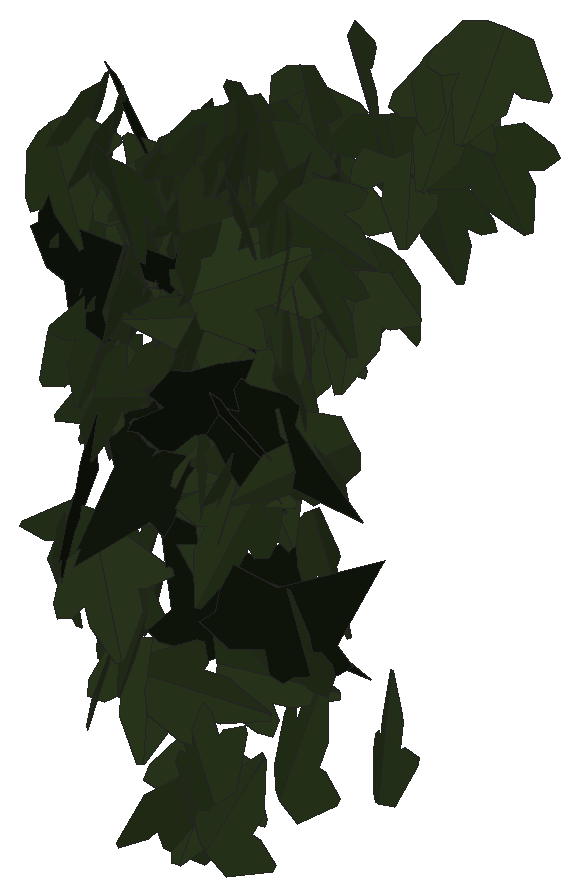
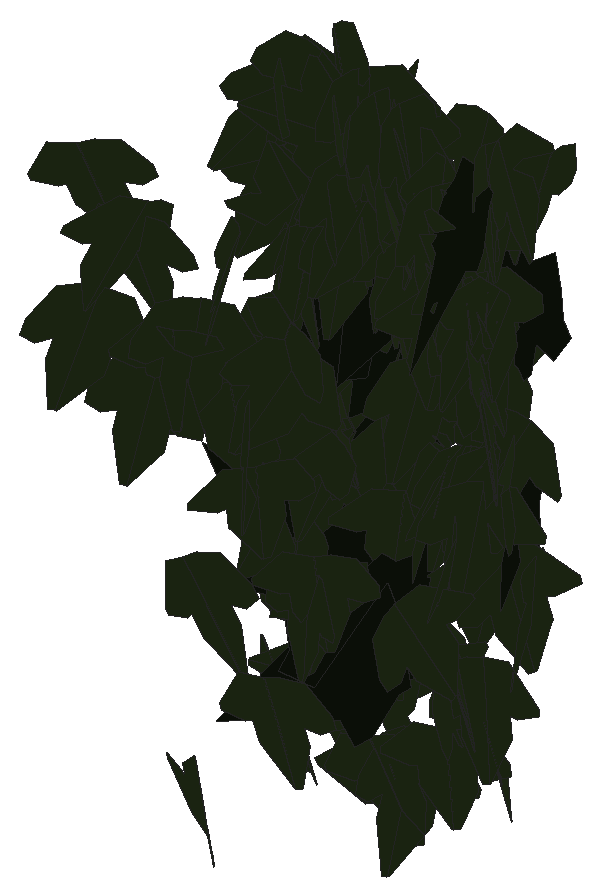
# SketchUp Ruby script. Lengths in inches.
U = 1.inch
M = Sketchup.active_model
def pt(a) = Geom::Point3d.new(a.map { |v| v * U })
def face(e, loops, mat)
  f = e.add_face(loops[0].map { |a| pt(a) })
  loops[1..].each { |l| e.add_face(l.map { |a| pt(a) }).erase! }
  f.material = f.back_material = mat if mat
  f
end
# faces: each face lists its corners as indices into pts; further lists are holes
def faces(e, pts, list, mat = nil) = list.each { |f| face(e, (f[0].is_a?(Array) ? f : [f]).map { |l| l.map { |i| pts[i] } }, mat) }
# xy, xz, yz: faces in a plane at the given z, y or x. An outline is a flat list of corners, or four numbers for a rectangle; further outlines are holes
def ring(l) = l.size == 4 ? [[l[0], l[1]], [l[2], l[1]], [l[2], l[3]], [l[0], l[3]]] : l.each_slice(2).to_a
def flat(e, list, mat, &to3) = list.each { |f| face(e, (f[0].is_a?(Array) ? f : [f]).map { |l| ring(l).map { |u, v| to3.(u, v) } }, mat) }
def xy(e, z, list, mat = nil) = flat(e, list, mat) { |x, y| [x, y, z] }
def xz(e, y, list, mat = nil) = flat(e, list, mat) { |x, z| [x, y, z] }
def yz(e, x, list, mat = nil) = flat(e, list, mat) { |y, z| [x, y, z] }
def lines(e, pts, list) = list.each { |a, b| e.add_line(pt(pts[a]), pt(pts[b])) }
# prism: a flat outline (further loops are holes) pulled along v
def prism(e, loops, v, mat = nil)
  f = face(e, loops, mat); d = Geom::Vector3d.new(v.map { |x| x * U })
  f.pushpull(f.normal.samedirection?(d) ? d.length : -d.length)
end
def box(e, o, s, mat = nil) = prism(e, [[o, [o[0] + s[0], o[1], o[2]], [o[0] + s[0], o[1] + s[1], o[2]], [o[0], o[1] + s[1], o[2]]]], [0, 0, s[2]], mat)
def at(x, y, z, deg = 0) = Geom::Transformation.translation(pt([x, y, z])) * Geom::Transformation.rotation(ORIGIN, Z_AXIS, deg.degrees)
def axes(o, x, y, z) = Geom::Transformation.new([*x, 0, *y, 0, *z, 0, *pt(o).to_a, 1])
def part(name) = M.definitions.add(name)
# library, detail: a bought-in or finely detailed component or shape, given as its bounding box
def library(name, o, s) = part(name).tap { |d| box(d.entities, o, s) }
def detail(e, o, s) = box(e.add_group.entities, o, s)
def put(e, d, t, mat = nil) = e.add_instance(d, t).tap { |i| i.material = mat if mat }
def group(e, t, mat = nil) = e.add_group.tap { |g| g.transformation = t; g.material = mat if mat }.entities
root = M.entities
M.materials.add("efeu1").color = [18, 25, 13]
M.materials.add("efeu2").color = [43, 57, 29]
c1 = part("ivyleaf_10")
p = [[0,0.5,-0.03],[-0.0625,2.02,-0.43],[-0.19,2.01,-0.46],[-0.54,1.05,-0.29],[-0.52,0.625,-0.18],[-0.83,0.76,-0.28],
  [-1.16,0.64,-0.33],[-1.15,0.33,-0.24],[-0.77,-0.39,0.02],[-0.3,-0.51,0.16],[0.04,-0.48,0.23],[-0.02,2.01,-0.4375],
  [-0.06,2.01,-0.43],[0.04,-0.49,0.23],[0.67,-0.49,0.14],[1.38,0.36,-0.2],[1.375,0.51,-0.24],[0.81,0.65,-0.19],
  [0.62,0.59,-0.15],[0.6,1.09,-0.28],[0.5,1.23,-0.31]]
faces(c1.entities,p,[[0,1,2,3,4,5,6,7,8,9,10],[11,12,0,13,14,15,16,17,18,19,20]],"efeu2")
c2 = part("ivyleaf_9")
p = [[1.54,2.16,1.25],[1.36,2.04,1.19],[-0.21,0.99,0.68],[-0.71,1.11,0.82],[-0.85,0.86,0.67],[-0.8,0.17,0.21],
  [-0.9,-0.01,0.1],[-0.67,-0.16,-0.02],[-0.08,-0.08,-0.05],[-0.03,-0.6,-0.4],[0.65,-0.88,-0.66],[0.83,-0.6,-0.49],
  [1.29,-0.42,-0.43],[1.8125,-0.07,-0.26],[1.21,0.44,0.15]]
faces(c2.entities,p,[[0,1,2,3,4,5,6,7,8,9,10,11,12,13,14]],"efeu1")
put(root,c1,axes([526.73,137.66,179.65],[0.34492,-0.55655,-0.19979],[-0.07334,0.18925,-0.65379],[0.58676,0.35081,0.03573]))
put(root,c1,axes([526.55,141.41,178.74],[0.59733,0.31347,-0.01678],[-0.01478,-0.00794,-0.67459],[-0.31357,0.59751,-0.00017]))
put(root,c1,axes([526.68,142.2,177.14],[0.6762,0.08427,-0.10291],[-0.10981,0.05281,-0.6783],[-0.07506,0.68194,0.06524]))
put(root,c1,axes([526.32,137.64,178.37],[0.22626,-0.32432,0.5422],[0.5291,-0.21748,-0.35088],[0.34528,0.54578,0.18237]))
put(root,c1,axes([526.96,136.28,176.09],[-0.253,0.3315,0.61469],[-0.38291,0.48091,-0.41696],[-0.58405,-0.45889,0.00709]))
put(root,c1,axes([526.73,137.78,178.06],[-0.4918,-0.46006,-0.10041],[0.12139,0.01642,-0.66977],[0.45497,-0.50167,0.07016]))
put(root,c1,axes([526.75,137.6,180.96],[0.06524,0.49402,0.48223],[-0.14861,0.48307,-0.47477],[-0.67417,-0.05868,0.15132]))
put(root,c1,axes([526.76,137.09,182.98],[0.15346,-0.69055,0.08481],[0.03468,-0.07915,-0.7072],[0.69488,0.15646,0.01657]))
put(root,c1,axes([526.82,141.39,178.37],[-0.62666,0.24212,0.03133],[-0.07654,-0.11287,-0.65856],[-0.23184,-0.6172,0.13272]))
put(root,c1,axes([526.55,137.1875,178.94],[-0.59271,-0.09398,-0.31926],[0.33268,-0.18537,-0.56305],[-0.00921,-0.6472,0.20763]))
put(root,c1,axes([526.95,137.45,175.16],[-0.65274,-0.09316,0.14039],[-0.13169,-0.06832,-0.65761],[0.10511,-0.66416,0.04796]))
put(root,c1,axes([526.91,139.04,176.77],[-0.16863,-0.55856,0.33637],[-0.03052,-0.34029,-0.58037],[0.65131,-0.16056,0.05989]))
put(root,c1,axes([526.89,137.52,181.05],[-0.2547,-0.64705,0.0378],[0.01176,-0.04522,-0.69483],[0.64804,-0.25349,0.02747]))
put(root,c1,axes([526.84,137.56,180.46],[0.20743,-0.65308,0.08528],[0.04003,-0.07674,-0.68508],[0.65741,0.21074,0.01481]))
put(root,c1,axes([527.0625,136.78,176.48],[-0.49027,-0.429,0.20414],[-0.13677,-0.15347,-0.65101],[0.45498,-0.50841,0.02427]))
put(root,c1,axes([526.79,138.34,177.59],[-0.29412,0.56067,-0.22412],[0.06235,-0.21976,-0.63159],[-0.60058,-0.29739,0.04419]))
put(root,c2,axes([526.875,137.77,182.61],[0.61826,-0.11639,-0.51976],[-0.4988,0.15278,-0.62754],[0.18681,0.79313,0.04461]))
put(root,c1,axes([526.79,136.36,182.55],[0.08652,0.72593,0.09804],[0.01904,0.09646,-0.73103],[-0.73227,0.08827,-0.00742]))
put(root,c1,axes([527,137.21,174.38],[0.38779,-0.55151,0.00364],[0.0023,-0.00284,-0.6742],[0.55152,0.3878,0.00025]))
put(root,c1,axes([527.37,137.79,177.8],[-0.54902,0.02235,-0.40135],[-0.40086,0.02003,0.54947],[0.02987,0.67978,-0.00299]))
put(root,c1,axes([527.1,137.05,182.73],[0.13063,-0.67134,-0.19616],[-0.03098,0.1938,-0.68391],[0.69873,0.13411,0.00635]))
put(root,c2,axes([526.62,136.75,180.27],[-0.08717,0.03371,0.78745],[0.44244,-0.65356,0.07696],[0.65227,0.44781,0.05303]))
put(root,c1,axes([527.11,137.1,179.79],[-0.09112,-0.67476,0.2638],[0.04855,-0.27097,-0.67632],[0.72286,-0.06685,0.07868]))
put(root,c2,axes([527.5,135.88,177.56],[-0.10562,0.10538,-0.81586],[-0.70882,0.4058,0.14418],[0.4175,0.71562,0.03838]))
put(root,c1,axes([527.22,137.16,181.21],[-0.53677,0.44477,0.03747],[-0.09582,-0.05758,-0.68909],[-0.43594,-0.53498,0.10532]))
put(root,c1,axes([527.17,137.8,175.63],[0.40583,-0.54322,0.02309],[0.01224,-0.01968,-0.67808],[0.54358,0.40601,-0.00197]))
put(root,c1,axes([527.17,137.51,181.125],[0.38421,-0.57202,-0.11484],[0.02053,0.15067,-0.68183],[0.58307,0.37162,0.09968]))
put(root,c1,axes([527.28,137.51,180.91],[0.546,-0.39262,-0.12601],[-0.1101,0.06268,-0.67238],[0.39737,0.55684,-0.01316]))
put(root,c1,axes([527.18,137.51,178.33],[-0.25362,-0.58125,-0.24503],[0.17351,0.18962,-0.62941],[0.60645,-0.29733,0.07761]))
put(root,c1,axes([527.67,137.58,181.76],[-0.4948,0.16819,0.44755],[-0.47688,-0.21967,-0.44469],[0.03418,-0.62998,0.27454]))
put(root,c1,axes([527.22,136.88,178.59],[-0.06189,-0.32946,-0.66162],[0.1774,0.63791,-0.33424],[0.71751,-0.18613,0.02557]))
put(root,c1,axes([527.1875,140.28,177.8125],[0.13331,0.65307,0.13137],[-0.00807,0.13555,-0.66565],[-0.6661,0.12906,0.03436]))
put(root,c1,axes([527.34,137.43,180.99],[-0.47146,0.51453,0.03959],[-0.03584,0.02085,-0.69775],[-0.5148,-0.47266,0.01232]))
put(root,c1,axes([527.27,137.69,180.78],[0.43151,0.50537,0.17621],[-0.00926,0.23337,-0.64661],[-0.53513,0.40347,0.15329]))
put(root,c1,axes([527.31,137.67,175.05],[0.16404,-0.57953,0.34818],[0.16922,-0.31168,-0.59851],[0.65456,0.22582,0.06747]))
put(root,c1,axes([527.46,137.33,180.51],[-0.01063,-0.70751,-0.00159],[0.00785,0.00147,-0.70754],[0.70746,-0.01064,0.00783]))
put(root,c1,axes([527.56,136.83,181.78],[-0.61387,0.27502,0.1835],[-0.16992,0.06952,-0.67263],[-0.28361,-0.63693,0.00582]))
put(root,c1,axes([527.53,137.39,181.24],[-0.17121,0.65872,0.16593],[-0.18514,0.1194,-0.665],[-0.65358,-0.20637,0.1449]))
put(root,c1,axes([527.62,136.93,181.9375],[-0.6839,-0.15676,0.04606],[-0.02555,-0.09317,-0.69647],[0.16137,-0.67908,0.08493]))
put(root,c1,axes([527.5,137.71,178.03],[-0.27325,0.62473,0.06912],[-0.02884,0.06282,-0.68187],[-0.62788,-0.27477,0.00124]))
put(root,c1,axes([527.57,137.5625,178.33],[-0.46744,0.48932,0.07753],[-0.05575,0.05397,-0.6767],[-0.49228,-0.47074,0.00301]))
put(root,c1,axes([527.4,140.95,181.3125],[-0.52133,-0.29503,-0.33284],[0.30593,0.13437,-0.5983],[0.32284,-0.60375,0.02949]))
put(root,c1,axes([527.43,137.53,174.08],[0.63628,0.29088,0.02502],[0.01821,0.02033,-0.69954],[-0.29138,0.63645,0.01091]))
put(root,c1,axes([527.6875,137.52,181.07],[-0.44649,-0.52236,-0.09133],[0.05124,0.07633,-0.6871],[0.5278,-0.4493,-0.01055]))
put(root,c1,axes([527.59,141.41,179.76],[0.44109,0.51607,-0.0565],[-0.0262,-0.05192,-0.67875],[-0.51849,0.44165,-0.01377]))
put(root,c1,axes([527.75,141.29,180.46],[0.18437,-0.56899,-0.32951],[-0.01701,0.33797,-0.59313],[0.6573,0.16834,0.07707]))
put(root,c1,axes([527.75,137.46,182.05],[-0.09166,-0.68778,-0.07675],[0.09267,0.06452,-0.6889],[0.68582,-0.10064,0.08283]))
put(root,c1,axes([527.59,136.32,176.2],[0.39292,0.54626,0.12166],[0.06463,0.10336,-0.67285],[-0.5559,0.39813,0.00776]))
put(root,c1,axes([527.48,140.87,181.74],[0.60239,-0.14425,0.30188],[0.32288,0.08776,-0.60237],[0.08766,0.66806,0.14431]))
put(root,c1,axes([527.69,137.48,181.51],[0.46198,0.50867,0.01464],[-0.00205,0.02164,-0.68696],[-0.50887,0.46171,0.01607]))
put(root,c1,axes([528.01,142.12,178.44],[0.5981,-0.03936,-0.35907],[-0.34125,0.16622,-0.58662],[0.11847,0.67751,0.12306]))
put(root,c1,axes([527.99,136.4,181.03],[0.08449,-0.49569,-0.54792],[-0.0309,0.54864,-0.5011],[0.73822,0.0797,0.04174]))
put(root,c1,axes([528.01,137.05,182.22],[-0.1309,0.51689,0.45995],[-0.22108,0.41232,-0.52628],[-0.65563,-0.24224,0.08564]))
put(root,c1,axes([527.98,136.23,182.59],[-0.6663,0.22065,-0.00081],[0.00029,-0.00172,-0.70188],[-0.22065,-0.6663,0.00154]))
put(root,c1,axes([527.79,137.11,181.95],[0.66696,0.2079,0.08704],[0.06322,0.08839,-0.69557],[-0.21634,0.66678,0.06506]))
put(root,c2,axes([528.3,136.8,178.02],[-0.75214,0.10885,-0.11708],[0.11551,-0.01931,-0.75997],[-0.11052,-0.76095,0.00254]))
put(root,c1,axes([528.01,137.41,179.35],[-0.32834,-0.56416,-0.21139],[0.15518,0.15342,-0.6505],[0.58213,-0.3591,0.05418]))
put(root,c1,axes([527.97,137.42,181.09],[0.65769,-0.35349,0.12885],[0.11257,-0.06272,-0.74666],[0.35901,0.66725,-0.00192]))
put(root,c1,axes([528.39,137.23,182.99],[0.02007,-0.70948,-0.05814],[-0.00658,0.05797,-0.70974],[0.71182,0.02054,-0.00492]))
put(root,c1,axes([528.29,137.5625,181.98],[0.36344,-0.52586,0.27284],[0.15528,-0.22435,-0.63923],[0.57171,0.39522,0.00017]))
put(root,c1,axes([528.33,137.42,181.4375],[-0.11255,0.67192,0.11822],[-0.02717,0.11531,-0.68123],[-0.6817,-0.11553,0.00764]))
put(root,c1,axes([528.73,137.06,178.15],[-0.50799,-0.28055,0.40562],[-0.33865,-0.22491,-0.57967],[0.35854,-0.60991,0.02718]))
put(root,c1,axes([528.51,137.29,182.07],[0.11156,-0.69891,0.03845],[-0.01508,-0.04133,-0.70744],[0.69981,0.11052,-0.02137]))
put(root,c1,axes([528.32,137.41,177.37],[0.4515,0.51129,0.06191],[0.04543,0.04246,-0.68208],[-0.51302,0.45374,-0.00592]))
put(root,c1,axes([528.63,137.1,182.55],[-0.67269,-0.16554,0.06589],[-0.06144,-0.02603,-0.69267],[0.16724,-0.6754,0.01055]))
put(root,c1,axes([528.45,137.29,182.82],[0.46192,-0.53007,0.10724],[0.1094,-0.04653,-0.70122],[0.52963,0.47192,0.05131]))
put(root,c2,axes([528.71,137.92,175.08],[0.359,0.22956,0.7152],[-0.6753,-0.24845,0.41872],[0.3289,-0.7607,0.07907]))
put(root,c1,axes([529.03,137.12,180.35],[0.16852,0.04351,-0.68613],[-0.68211,-0.07779,-0.17247],[-0.08601,0.70223,0.02341]))
put(root,c1,axes([528.54,140.84,182.65],[-0.39616,0.57073,-0.00023],[-0.00159,-0.00138,-0.69474],[-0.57072,-0.39616,0.00209]))
put(root,c1,axes([528.77,137.3,183.05],[-0.08629,-0.70447,0.00916],[0.00164,-0.00943,-0.70973],[0.70453,-0.08626,0.00278]))
put(root,c2,axes([528.57,136.79,181.1875],[0.68322,0.38247,-0.13387],[-0.11502,-0.06859,-0.78298],[-0.38856,0.69282,-0.00361]))
put(root,c1,axes([528.83,136.83,180.18],[0.22584,-0.64894,-0.08842],[-0.03894,0.08006,-0.68703],[0.65377,0.22894,-0.01038]))
put(root,c1,axes([528.8125,136.54,172.98],[-0.28899,-0.67888,-0.2729],[0.1037,0.25245,-0.73782],[0.72429,-0.30702,-0.00325]))
put(root,c1,axes([528.91,141.08,181.52],[-0.59318,-0.39996,-0.06692],[0.05994,0.0308,-0.71538],[0.40106,-0.59615,0.00794]))
put(root,c1,axes([528.91,137.22,181.3],[0.1838,-0.67422,-0.05252],[-0.01036,0.05161,-0.69881],[0.67618,0.18406,0.00357]))
put(root,c1,axes([528.93,137.48,182.82],[0.14098,-0.67536,0.11177],[0.00888,-0.1123,-0.68978],[0.68449,0.14056,-0.01407]))
put(root,c1,axes([528.97,137.3,183.37],[-0.34963,-0.61331,-0.04929],[0.02931,0.04003,-0.70594],[0.61459,-0.35082,0.00562]))
put(root,c2,axes([528.375,137.96,175.37],[0.7729,0.01068,0.29831],[0.2983,0.00241,-0.77297],[-0.01083,0.82846,-0.0016]))
put(root,c1,axes([528.84,137.58,181.84],[-0.47746,-0.39412,-0.31386],[0.24316,0.19846,-0.61911],[0.44126,-0.53581,0.00156]))
put(root,c1,axes([528.98,137.02,173.18],[0.70863,0.13646,-0.15114],[-0.14773,-0.03209,-0.72164],[-0.14014,0.72386,-0.0035]))
put(root,c1,axes([529.05,137.6,182.18],[-0.30074,-0.62446,-0.04999],[0.07695,0.01821,-0.69039],[0.62172,-0.30432,0.06127]))
put(root,c1,axes([528.6,138.76,178.88],[0.45747,-0.00612,0.51026],[0.50443,0.10904,-0.45094],[-0.07716,0.67658,0.07729]))
put(root,c1,axes([528.72,137.21,178.53],[0.14131,-0.3027,0.65661],[0.50727,-0.43522,-0.30981],[0.5152,0.51155,0.12495]))
put(root,c1,axes([529.1,136.74,180.68],[0.26251,-0.6428,0.0458],[0.00443,-0.04765,-0.6942],[0.64441,0.26218,-0.01388]))
put(root,c1,axes([529.16,137.5,181.28],[-0.24277,-0.61321,-0.22742],[0.06794,0.21763,-0.65932],[0.65048,-0.25159,-0.01601]))
put(root,c1,axes([529.47,136.375,173.51],[0.54477,-0.07923,0.49181],[-0.48824,0.05969,0.55044],[-0.09885,-0.7315,-0.00835]))
put(root,c1,axes([528.72,136.45,174.66],[0.11488,-0.02257,0.68917],[0.56067,0.40976,-0.08004],[-0.40139,0.56591,0.08545]))
put(root,c1,axes([529.12,141.22,181.18],[0.63077,0.27627,0.02283],[0.00454,0.04644,-0.68742],[-0.27717,0.62947,0.0407]))
put(root,c1,axes([529.27,137.44,183.12],[0.24781,-0.65475,-0.05712],[0.01196,0.06553,-0.69924],[0.65713,0.24572,0.03427]))
put(root,c1,axes([529.27,137.17,178.06],[0.5292,0.40547,-0.18058],[-0.13404,-0.12189,-0.66652],[-0.42314,0.54572,-0.0147]))
put(root,c1,axes([529.37,137.17,178.23],[0.21838,-0.68765,0.04104],[0.00511,-0.04144,-0.72145],[0.68885,0.21831,-0.00766]))
put(root,c1,axes([529.51,136.85,182.57],[-0.49934,0.43351,0.23528],[-0.21035,0.11567,-0.65954],[-0.44614,-0.53973,0.04763]))
put(root,c2,axes([529.16,136.65,179.24],[0.74295,-0.01466,-0.22358],[-0.22356,0.0034,-0.74309],[0.01502,0.77585,-0.00097]))
put(root,c1,axes([529.38,139.69,179.66],[0.41661,0.54406,-0.10376],[-0.09367,-0.05876,-0.68418],[-0.54589,0.4253,0.03821]))
put(root,c1,axes([529.47,141.37,180.53],[-0.7037,-0.07647,-0.06876],[0.07072,-0.01463,-0.7075],[0.07466,-0.7069,0.02208]))
put(root,c1,axes([529.49,135.85,182.47],[0.14855,-0.25111,-0.68556],[0.0361,0.70127,-0.24904],[0.72921,0.01644,0.15199]))
put(root,c2,axes([529.15,135.89,179.49],[0.50713,0.41395,0.46497],[0.36829,0.28402,-0.65454],[-0.50191,0.62666,-0.01049]))
put(root,c1,axes([529.54,137.09,177.5],[-0.23531,-0.55966,0.43975],[0.04295,-0.47348,-0.57961],[0.71046,-0.15674,0.18069]))
put(root,c1,axes([529.66,136.98,183.65],[0.44739,-0.34329,-0.46306],[-0.23607,0.42563,-0.54363],[0.52587,0.48313,0.1499]))
put(root,c1,axes([529.39,137.5625,177.93],[0.10124,0.65541,0.20969],[0.01264,0.21014,-0.66292],[-0.68802,0.10031,0.01868]))
put(root,c1,axes([529.02,137.59,174.49],[-0.03097,-0.02575,0.73455],[0.65848,0.32566,0.03918],[-0.32655,0.65914,0.00934]))
put(root,c1,axes([529.79,137.13,178.43],[-0.50417,-0.47222,0.0787],[-0.06268,-0.0482,-0.69074],[0.47461,-0.508,-0.00762]))
put(root,c1,axes([529.42,136.67,172.5],[0.63569,-0.18503,-0.31988],[0.30604,-0.09313,0.66206],[-0.20712,-0.70551,-0.00351]))
put(root,c1,axes([529.52,136.41,181.3125],[0.36954,-0.09053,-0.64841],[0.65118,0.12791,0.35326],[0.06778,-0.73528,0.14129]))
put(root,c1,axes([529.95,137.41,180.9],[0.11904,0.69325,0.00408],[-0.00134,0.00437,-0.70339],[-0.69326,0.11903,0.00206]))
put(root,c1,axes([530.05,140.95,182.51],[0.71908,-0.00361,-0.09168],[-0.09171,-0.0063,-0.71906],[0.00278,0.72487,-0.0067]))
put(root,c1,axes([529.9,141.15,182.83],[0.19199,0.63545,0.29134],[0.09119,0.27678,-0.66379],[-0.69308,0.21244,-0.00663]))
put(root,c1,axes([529.55,137.5,182.71],[0.01158,-0.07304,0.69553],[0.67728,0.17457,0.00705],[-0.17432,0.67337,0.07361]))
put(root,c1,axes([530.01,137.31,183.38],[-0.64839,0.09629,-0.2497],[0.23226,-0.12268,-0.65042],[-0.13296,-0.6839,0.08152]))
put(root,c1,axes([530.2,137.375,181.17],[-0.36564,0.60279,-0.01072],[-0.03989,-0.0367,-0.70301],[-0.60156,-0.36396,0.05313]))
put(root,c1,axes([529.97,137.6,173.2],[0.71266,-0.41458,-0.15108],[0.13809,-0.06302,0.82434],[-0.41909,-0.72577,0.01472]))
put(root,c1,axes([530.63,136.76,180.1875],[-0.29072,0.21104,0.62694],[-0.57455,0.25883,-0.35355],[-0.32784,-0.64076,0.06367]))
put(root,c1,axes([530.09,137.32,181.17],[0.6586,0.19342,-0.16119],[0.12137,0.1516,0.67782],[0.2206,-0.66087,0.10831]))
put(root,c1,axes([530.35,137.18,175.22],[-0.70824,0.0057,0.0145],[0.01444,-0.00699,0.70823],[0.00584,0.70835,0.00687]))
put(root,c1,axes([530.35,139.16,172.61],[0.58549,-0.32915,0.24817],[-0.21662,0.12111,0.67167],[-0.35073,-0.62428,-0.00055]))
put(root,c1,axes([530.29,141.58,181.46],[-0.52822,-0.4412,-0.21337],[0.22147,0.06495,-0.68259],[0.43718,-0.56597,0.08799]))
put(root,c1,axes([530.73,137.11,178.75],[-0.54459,0.07206,0.44525],[-0.43839,0.07964,-0.54909],[-0.1061,-0.69892,-0.01666]))
put(root,c1,axes([530.43,137.05,183.04],[0.12945,-0.69706,0.04803],[0.00335,-0.04823,-0.70896],[0.6987,0.12938,-0.0055]))
put(root,c1,axes([530.05,137.99,176.82],[0.49626,-0.29985,0.41047],[0.45863,0.01676,-0.54226],[0.2192,0.6438,0.20529]))
put(root,c2,axes([529.89,136.59,179.29],[0.02007,0.03924,-0.75868],[0.61975,0.43809,0.03906],[0.43937,-0.61974,-0.02043]))
put(root,c1,axes([530.62,136.58,182.35],[0.32716,-0.42733,-0.45695],[-0.18989,0.42351,-0.53201],[0.59612,0.36943,0.08132]))
put(root,c2,axes([530.12,136.85,175.65],[-0.12115,-0.11905,0.76279],[0.77116,-0.05525,0.11386],[0.03658,0.77038,0.12604]))
put(root,c1,axes([530.53,137.3,181.6],[-0.66073,0.11765,-0.22453],[0.21957,-0.04762,-0.67108],[-0.12667,-0.69622,0.00796]))
put(root,c1,axes([530.96,137.125,178.87],[-0.11111,-0.26039,0.66905],[-0.28293,-0.60634,-0.28297],[0.65983,-0.30384,-0.00867]))
put(root,c1,axes([530.74,141.07,183.43],[0.64195,0.24323,-0.15892],[-0.14114,-0.07583,-0.68618],[-0.25396,0.65696,-0.02036]))
put(root,c1,axes([530.62,136.9375,182.65],[-0.43124,-0.2955,-0.48237],[0.40322,0.26485,-0.52272],[0.39676,-0.59035,0.00694]))
